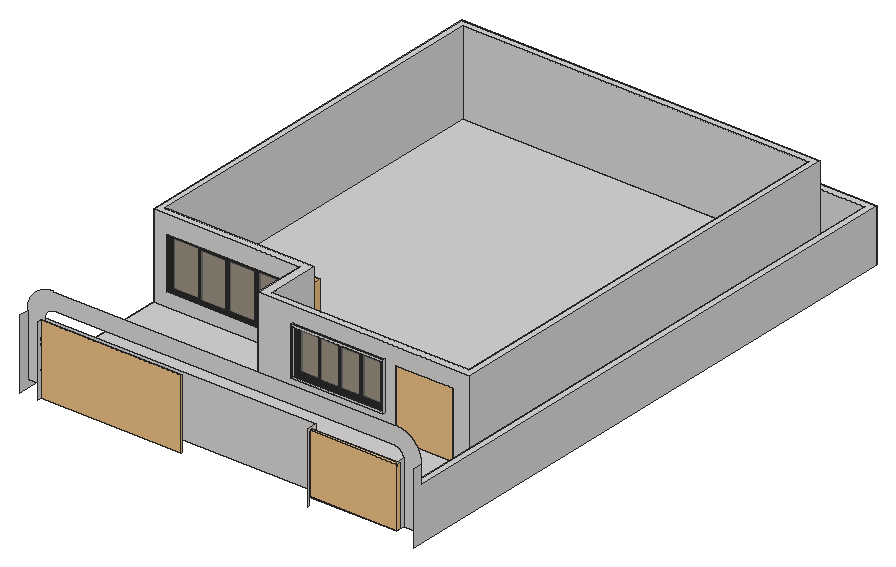
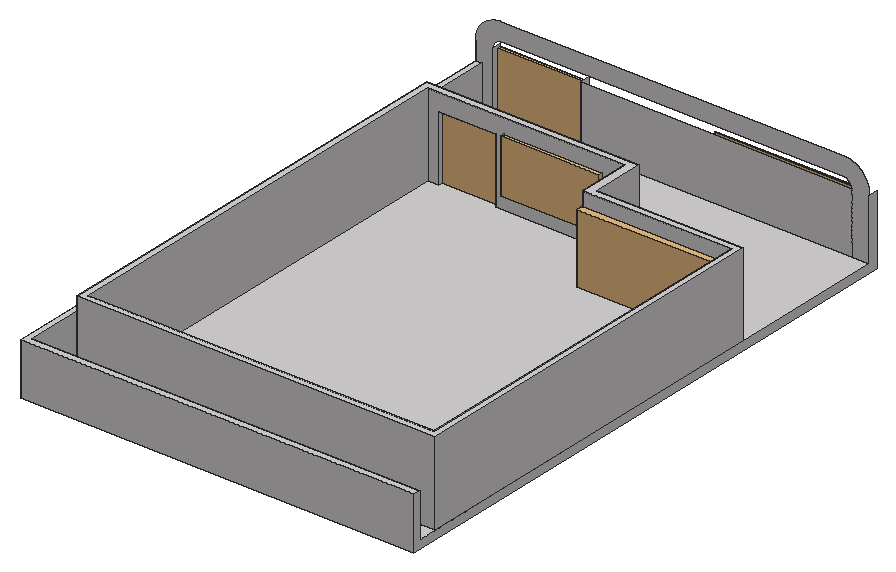
# SketchUp Ruby script. Lengths in inches.
U = 1.inch
M = Sketchup.active_model
def pt(a) = Geom::Point3d.new(a.map { |v| v * U })
def face(e, loops, mat)
  f = e.add_face(loops[0].map { |a| pt(a) })
  loops[1..].each { |l| e.add_face(l.map { |a| pt(a) }).erase! }
  f.material = f.back_material = mat if mat
  f
end
# faces: each face lists its corners as indices into pts; further lists are holes
def faces(e, pts, list, mat = nil) = list.each { |f| face(e, (f[0].is_a?(Array) ? f : [f]).map { |l| l.map { |i| pts[i] } }, mat) }
# xy, xz, yz: faces in a plane at the given z, y or x. An outline is a flat list of corners, or four numbers for a rectangle; further outlines are holes
def ring(l) = l.size == 4 ? [[l[0], l[1]], [l[2], l[1]], [l[2], l[3]], [l[0], l[3]]] : l.each_slice(2).to_a
def flat(e, list, mat, &to3) = list.each { |f| face(e, (f[0].is_a?(Array) ? f : [f]).map { |l| ring(l).map { |u, v| to3.(u, v) } }, mat) }
def xy(e, z, list, mat = nil) = flat(e, list, mat) { |x, y| [x, y, z] }
def xz(e, y, list, mat = nil) = flat(e, list, mat) { |x, z| [x, y, z] }
def yz(e, x, list, mat = nil) = flat(e, list, mat) { |y, z| [x, y, z] }
def lines(e, pts, list) = list.each { |a, b| e.add_line(pt(pts[a]), pt(pts[b])) }
# prism: a flat outline (further loops are holes) pulled along v
def prism(e, loops, v, mat = nil)
  f = face(e, loops, mat); d = Geom::Vector3d.new(v.map { |x| x * U })
  f.pushpull(f.normal.samedirection?(d) ? d.length : -d.length)
end
def box(e, o, s, mat = nil) = prism(e, [[o, [o[0] + s[0], o[1], o[2]], [o[0] + s[0], o[1] + s[1], o[2]], [o[0], o[1] + s[1], o[2]]]], [0, 0, s[2]], mat)
def at(x, y, z, deg = 0) = Geom::Transformation.translation(pt([x, y, z])) * Geom::Transformation.rotation(ORIGIN, Z_AXIS, deg.degrees)
def axes(o, x, y, z) = Geom::Transformation.new([*x, 0, *y, 0, *z, 0, *pt(o).to_a, 1])
def part(name) = M.definitions.add(name)
# library, detail: a bought-in or finely detailed component or shape, given as its bounding box
def library(name, o, s) = part(name).tap { |d| box(d.entities, o, s) }
def detail(e, o, s) = box(e.add_group.entities, o, s)
def put(e, d, t, mat = nil) = e.add_instance(d, t).tap { |i| i.material = mat if mat }
def group(e, t, mat = nil) = e.add_group.tap { |g| g.transformation = t; g.material = mat if mat }.entities
root = M.entities
M.materials.add("T METAL").color = [42, 41, 39]
M.materials.add("[Quartz Light Brown]").color = [215, 212, 212]
M.materials.add("[Terrazzo Tile Light]").color = [219, 217, 210]
M.materials.add("[Translucent_Glass_Gray]").color = [128, 128, 128]
M.materials["[Translucent_Glass_Gray]"].alpha = 0.5
M.materials.add("[Wood Cherry Original]").color = [152, 86, 42]
c1 = library("cong+trinh+1",[72.29,25.93,6.78],[125.98,5.19,98.43])
c2 = library("Group\#56",[0,-0.5,0],[192,0.5,96])
c3 = library("Garniza_zaclona",[1.52,0,0],[127.96,8.15,78.72])
c4 = part("Window frame")
prism(c4.entities,[[[0,70.87,0],[0,0,0],[0,0,47.24],[0,70.87,47.24]],[[0,1.97,1.97],[0,68.9,1.97],[0,68.9,45.28],[0,1.97,45.28]]],[7.875,0,0])
c5 = part("Window sash")
xy(c5.entities,0,[[0,0,3.9375,16.73]])
xy(c5.entities,0.98,[[0,0.98,1.77,15.75],[1.77,0.98,2.85,15.75],[2.85,0.98,3.9375,15.75]])
xy(c5.entities,42.32,[[0,0.98,1.77,15.75],[1.77,0.98,2.85,15.75],[2.85,0.98,3.9375,15.75]])
xy(c5.entities,43.31,[[0,0,3.9375,16.73]])
xz(c5.entities,0,[[0,0,3.9375,43.31]])
xz(c5.entities,0.98,[[0,0.98,1.77,42.32],[1.77,0.98,2.85,42.32],[2.85,0.98,3.9375,42.32]])
xz(c5.entities,15.75,[[0,0.98,1.77,42.32],[1.77,0.98,2.85,42.32],[2.85,0.98,3.9375,42.32]])
xz(c5.entities,16.73,[[0,0,3.9375,43.31]])
yz(c5.entities,0,[[[0,0,16.73,43.31],[0.98,0.98,15.75,42.32]]])
yz(c5.entities,1.77,[[0.98,0.98,15.75,42.32]],"[Translucent_Glass_Gray]")
yz(c5.entities,2.85,[[0.98,0.98,15.75,42.32]],"[Translucent_Glass_Gray]")
yz(c5.entities,3.9375,[[[0,0,16.73,43.31],[0.98,0.98,15.75,42.32]]])
c6 = part("simple+window")
p = [[0,68.9,1.97],[0,35.43,1.97]]
lines(c6.entities,p,[[0,1]])
put(c6.entities,c4,at(0,0,0))
put(c6.entities,c5,axes([1.14,52.17,1.97],[0.71,0,0],[0,1,0],[0,0,1]))
put(c6.entities,c5,axes([1.14,1.97,1.97],[0.71,0,0],[0,1,0],[0,0,1]))
put(c6.entities,c5,axes([3.9375,18.7,1.97],[0.71,0,0],[0,1,0],[0,0,1]))
put(c6.entities,c5,axes([3.9375,35.43,1.97],[0.71,0,0],[0,1,0],[0,0,1]))
c7 = library("Elegant door(double)",[38.88,29.07,0],[76.71,4.33,84.81])
c8 = library("SHOWER+CURTAIN",[-76.11,-2.58,2.78],[135.11,4.99,73.24])
xy(root,0,[[396,38,516,38,516,50,531,50,531,821,0,821,0,50,396,50]],"[Quartz Light Brown]")
xy(root,60,[[531,50,540,50,540,830,0,830,0,821,531,821]],"[Quartz Light Brown]")
xz(root,44,[[24,-12,216,84]],"[Quartz Light Brown]")
xz(root,50,[[0,0,0,84.57,0.03,85.41,0.04,85.7,0.05,85.98,0.11,86.82,0.13,87.11,0.16,87.39,0.1875,87.67,0.22,87.95,0.28,88.51,0.44,89.63,0.49,89.91,0.54,90.1875,0.59,90.47,0.64,90.75,0.69,91.02,0.81,91.58,0.87,91.85,0.93,92.13,0.99,92.4,1.0625,92.68,1.2,93.23,1.28,93.5,1.35,93.77,1.51,94.31,1.59,94.59,1.68,94.86,1.76,95.125,1.85,95.39,2.03,95.93,2.13,96.19,2.23,96.46,2.32,96.73,2.42,96.99,2.53,97.25,2.63,97.51,2.74,97.78,3.07,98.56,3.1875,98.81,3.31,99.07,3.43,99.33,3.55,99.58,3.67,99.84,3.8,100.09,3.92,100.34,4.05,100.6,4.18,100.85,4.32,101.09,4.45,101.34,4.73,101.84,4.87,102.08,5.01,102.33,5.16,102.57,5.3,102.81,5.6,103.29,5.76,103.53,5.91,103.76,6.23,104.24,6.38,104.47,6.55,104.7,6.71,104.93,7.04,105.39,7.21,105.62,7.55,106.06,7.73,106.29,7.9,106.51,8.26,106.95,8.44,107.16,8.625,107.38,8.81,107.59,9,107.81,9.18,108.02,9.375,108.23,9.5625,108.4375,9.76,108.64,9.95,108.85,10.15,109.05,10.35,109.26,10.54,109.46,10.74,109.65,10.95,109.85,11.15,110.05,11.36,110.24,11.5625,110.4375,11.77,110.625,11.98,110.82,12.19,111,12.41,111.19,12.62,111.375,12.84,111.56,13.05,111.74,13.49,112.1,13.71,112.27,13.94,112.45,14.38,112.79,14.61,112.96,15.07,113.29,15.3,113.45,15.53,113.62,15.76,113.77,16.24,114.09,16.47,114.24,16.71,114.4,17.19,114.7,17.43,114.84,17.67,114.99,17.92,115.13,18.16,115.27,18.66,115.55,18.91,115.68,19.15,115.82,19.4,115.95,19.66,116.08,19.91,116.2,20.16,116.33,20.42,116.45,20.67,116.57,20.93,116.69,21.19,116.8125,21.44,116.93,22.22,117.26,22.49,117.37,22.75,117.47,23.01,117.58,23.27,117.68,23.54,117.77,23.81,117.87,24.07,117.97,24.61,118.15,24.875,118.24,25.14,118.32,25.41,118.41,25.69,118.49,26.23,118.65,26.5,118.72,26.77,118.8,27.32,118.9375,27.6,119.01,27.87,119.07,28.15,119.13,28.42,119.19,28.98,119.31,29.25,119.36,29.53,119.41,29.8125,119.46,30.09,119.51,30.37,119.56,31.49,119.72,32.05,119.78,32.33,119.8125,32.61,119.84,32.89,119.87,33.18,119.89,34.02,119.95,34.3,119.96,34.59,119.97,35.43,120,504.57,120,505.41,119.97,505.7,119.96,505.98,119.95,506.82,119.89,507.11,119.87,507.39,119.84,507.67,119.8125,507.95,119.78,508.51,119.72,509.63,119.56,509.91,119.51,510.1875,119.46,510.47,119.41,510.75,119.36,511.02,119.31,511.58,119.19,511.85,119.13,512.13,119.07,512.4,119.01,512.68,118.9375,513.23,118.8,513.5,118.72,513.77,118.65,514.31,118.49,514.59,118.41,514.86,118.32,515.125,118.24,515.39,118.15,515.93,117.97,516.19,117.87,516.46,117.77,516.73,117.68,516.99,117.58,517.25,117.47,517.51,117.37,517.78,117.26,518.56,116.93,518.81,116.8125,519.07,116.69,519.33,116.57,519.58,116.45,519.84,116.33,520.09,116.2,520.34,116.08,520.6,115.95,520.85,115.82,521.09,115.68,521.34,115.55,521.84,115.27,522.08,115.13,522.33,114.99,522.57,114.84,522.81,114.7,523.29,114.4,523.53,114.24,523.76,114.09,524.24,113.77,524.47,113.62,524.7,113.45,524.93,113.29,525.39,112.96,525.62,112.79,526.06,112.45,526.29,112.27,526.51,112.1,526.95,111.74,527.16,111.56,527.38,111.375,527.59,111.19,527.81,111,528.02,110.82,528.23,110.625,528.4375,110.4375,528.64,110.24,528.85,110.05,529.05,109.85,529.26,109.65,529.46,109.46,529.65,109.26,529.85,109.05,530.05,108.85,530.24,108.64,530.4375,108.4375,530.625,108.23,530.82,108.02,531,107.81,531.19,107.59,531.375,107.38,531.56,107.16,531.74,106.95,532.1,106.51,532.27,106.29,532.45,106.06,532.79,105.62,532.96,105.39,533.29,104.93,533.45,104.7,533.62,104.47,533.77,104.24,534.09,103.76,534.24,103.53,534.4,103.29,534.7,102.81,534.84,102.57,534.99,102.33,535.13,102.08,535.27,101.84,535.55,101.34,535.68,101.09,535.82,100.85,535.95,100.6,536.08,100.34,536.2,100.09,536.33,99.84,536.45,99.58,536.57,99.33,536.69,99.07,536.8125,98.81,536.93,98.56,537.26,97.78,537.37,97.51,537.47,97.25,537.58,96.99,537.68,96.73,537.77,96.46,537.87,96.19,537.97,95.93,538.15,95.39,538.24,95.125,538.32,94.86,538.41,94.59,538.49,94.31,538.65,93.77,538.72,93.5,538.8,93.23,538.9375,92.68,539.01,92.4,539.07,92.13,539.13,91.85,539.19,91.58,539.31,91.02,539.36,90.75,539.41,90.47,539.46,90.1875,539.51,89.91,539.56,89.63,539.72,88.51,539.78,87.95,539.8125,87.67,539.84,87.39,539.87,87.11,539.89,86.82,539.95,85.98,539.96,85.7,539.97,85.41,540,84.57,540,60,531,60,531,0,516,0,516,84.28,515.99,84.375,515.99,84.57,515.98,84.66,515.98,84.75,515.97,84.85,515.96,84.94,515.96,85.04,515.95,85.13,515.9375,85.22,515.93,85.32,515.91,85.5,515.89,85.6,515.87,85.78,515.85,85.88,515.84,85.97,515.82,86.0625,515.8,86.16,515.79,86.25,515.75,86.43,515.73,86.53,515.65,86.89,515.62,86.98,515.6,87.08,515.57,87.17,515.55,87.26,515.52,87.35,515.5,87.4375,515.47,87.53,515.32,87.98,515.29,88.06,515.23,88.24,515.19,88.33,515.16,88.42,515.12,88.5,515.09,88.59,515.01,88.77,514.98,88.85,514.9375,88.9375,514.9,89.02,514.86,89.11,514.82,89.19,514.78,89.28,514.73,89.36,514.69,89.45,514.65,89.53,514.61,89.62,514.5625,89.7,514.52,89.78,514.47,89.86,514.42,89.95,514.33,90.11,514.28,90.1875,514.23,90.27,513.98,90.67,513.92,90.75,513.87,90.82,513.82,90.9,513.76,90.98,513.71,91.05,513.65,91.13,513.6,91.21,513.48,91.35,513.42,91.43,513.37,91.5,513.31,91.58,513.25,91.65,513.0625,91.86,513,91.9375,512.9375,92.01,512.8125,92.15,512.75,92.21,512.68,92.28,512.62,92.35,512.55,92.42,512.49,92.49,512.42,92.55,512.35,92.62,512.28,92.68,512.21,92.75,512.15,92.8125,512.01,92.9375,511.9375,93,511.86,93.0625,511.65,93.25,511.58,93.31,511.5,93.37,511.43,93.42,511.35,93.48,511.21,93.6,511.13,93.65,511.05,93.71,510.98,93.76,510.9,93.82,510.82,93.87,510.75,93.92,510.67,93.98,510.27,94.23,510.1875,94.28,510.11,94.33,509.95,94.42,509.86,94.47,509.78,94.52,509.7,94.5625,509.62,94.61,509.53,94.65,509.45,94.69,509.36,94.73,509.28,94.78,509.19,94.82,509.11,94.86,509.02,94.9,508.9375,94.9375,508.85,94.98,508.77,95.01,508.59,95.09,508.5,95.12,508.42,95.16,508.33,95.19,508.24,95.23,508.06,95.29,507.98,95.32,507.53,95.47,507.4375,95.5,507.35,95.52,507.26,95.55,507.17,95.57,507.08,95.6,506.98,95.62,506.89,95.65,506.53,95.73,506.43,95.75,506.25,95.79,506.16,95.8,506.0625,95.82,505.97,95.84,505.88,95.85,505.78,95.87,505.6,95.89,505.5,95.91,505.32,95.93,505.22,95.9375,505.13,95.95,505.04,95.96,504.94,95.96,504.85,95.97,504.75,95.98,504.66,95.98,504.57,95.99,504.375,95.99,504.28,96,35.72,96,35.625,95.99,35.43,95.99,35.34,95.98,35.25,95.98,35.15,95.97,35.06,95.96,34.96,95.96,34.87,95.95,34.78,95.9375,34.68,95.93,34.5,95.91,34.4,95.89,34.22,95.87,34.12,95.85,34.03,95.84,33.9375,95.82,33.84,95.8,33.75,95.79,33.57,95.75,33.47,95.73,33.11,95.65,33.02,95.62,32.92,95.6,32.83,95.57,32.74,95.55,32.65,95.52,32.5625,95.5,32.47,95.47,32.02,95.32,31.94,95.29,31.76,95.23,31.67,95.19,31.58,95.16,31.5,95.12,31.41,95.09,31.23,95.01,31.15,94.98,31.0625,94.9375,30.98,94.9,30.89,94.86,30.81,94.82,30.72,94.78,30.64,94.73,30.55,94.69,30.47,94.65,30.38,94.61,30.3,94.5625,30.22,94.52,30.14,94.47,30.05,94.42,29.89,94.33,29.8125,94.28,29.73,94.23,29.33,93.98,29.25,93.92,29.18,93.87,29.1,93.82,29.02,93.76,28.95,93.71,28.87,93.65,28.79,93.6,28.65,93.48,28.57,93.42,28.5,93.37,28.42,93.31,28.35,93.25,28.14,93.0625,28.0625,93,27.99,92.9375,27.85,92.8125,27.79,92.75,27.72,92.68,27.65,92.62,27.58,92.55,27.51,92.49,27.45,92.42,27.38,92.35,27.32,92.28,27.25,92.21,27.1875,92.15,27.0625,92.01,27,91.9375,26.9375,91.86,26.75,91.65,26.69,91.58,26.63,91.5,26.58,91.43,26.52,91.35,26.4,91.21,26.35,91.13,26.29,91.05,26.24,90.98,26.18,90.9,26.13,90.82,26.08,90.75,26.02,90.67,25.77,90.27,25.72,90.1875,25.67,90.11,25.58,89.95,25.53,89.86,25.48,89.78,25.4375,89.7,25.39,89.62,25.35,89.53,25.31,89.45,25.27,89.36,25.22,89.28,25.18,89.19,25.14,89.11,25.1,89.02,25.0625,88.9375,25.02,88.85,24.99,88.77,24.91,88.59,24.88,88.5,24.84,88.42,24.81,88.33,24.77,88.24,24.71,88.06,24.68,87.98,24.53,87.53,24.5,87.4375,24.48,87.35,24.45,87.26,24.43,87.17,24.4,87.08,24.38,86.98,24.35,86.89,24.27,86.53,24.25,86.43,24.21,86.25,24.2,86.16,24.18,86.0625,24.16,85.97,24.15,85.88,24.13,85.78,24.11,85.6,24.09,85.5,24.07,85.32,24.0625,85.22,24.05,85.13,24.04,85.04,24.04,84.94,24.03,84.85,24.02,84.75,24.02,84.66,24.01,84.57,24.01,84.375,24,84.28,24,0],[24,0,396,84]],"[Quartz Light Brown]")
xz(root,821,[[0,0,531,60]],"[Quartz Light Brown]")
xz(root,830,[[0,-12,540,60]],"[Quartz Light Brown]")
yz(root,0,[[38,-12,38,84,50,84,50,0,821,0,821,60,830,60,830,-12]],"[Quartz Light Brown]")
yz(root,24,[[38,-12,44,84]],"[Quartz Light Brown]")
yz(root,396,[[36,-12,38,-12,38,0,50,0,50,84,36,84]],"[Terrazzo Tile Light]")
yz(root,516,[[38,0,50,84]],"[Quartz Light Brown]")
yz(root,531,[[50,0,821,60]],"[Quartz Light Brown]")
yz(root,540,[[38,-12,830,-12,830,60,50,60,50,84,38,84]],"[Quartz Light Brown]")
put(root,c1,axes([327.15,16.74,-5.59],[0.9525,0,0],[0,0.85,0],[0,0,0.8245]),"[Quartz Light Brown]")
put(root,c2,at(24,44,-12),"[Wood Cherry Original]")
put(root,c3,axes([9,275,0],[1.58151,0,0],[0,1.1771,0],[0,0,1.20432]),"[Quartz Light Brown]")
g1 = group(root,at(0,194,0),"[Quartz Light Brown]")
xy(g1,0,[[201,0,201,72,0,72,0,600,492,600,492,0,468,0,468,9,483,9,483,591,9,591,9,81,213,81,213,9,390,9,390,0]])
xy(g1,18,[[18,72,183,81]])
xy(g1,27,[[249,-3,375,0]])
xy(g1,29.5,[[251.5,-3,372.5,0]])
xy(g1,30,[[252,0,372,9]])
xy(g1,90,[[252,0,372,9],[390,0,468,9],[18,72,183,81]])
xy(g1,90.5,[[251.5,-3,372.5,0]])
xy(g1,93,[[249,-3,375,0]])
xy(g1,114,[[[201,0,492,0,492,600,0,600,0,72,201,72],[213,9,213,81,9,81,9,591,483,591,483,9]]])
xz(g1,-3,[[[249,27,375,93],[251.5,29.5,372.5,90.5]]])
xz(g1,0,[[[201,0,390,0,390,90,468,90,468,0,492,0,492,114,201,114],[249,27,375,93]],[[251.5,29.5,372.5,90.5],[252,30,372,90]],[372.5,29.5,373,91.5],[373,29.5,373.5,91.5]])
xz(g1,9,[[[213,0,213,114,483,114,483,0,468,0,468,90,390,90,390,0],[252,30,372,90]]])
xz(g1,72,[[[0,0,201,114],[18,18,183,90]]])
xz(g1,81,[[[9,0,213,114],[18,18,183,90]]])
xz(g1,591,[[9,0,483,114]])
xz(g1,600,[[0,0,492,114]])
yz(g1,0,[[72,0,600,114]])
yz(g1,9,[[81,0,591,114]])
yz(g1,18,[[72,18,81,90]])
yz(g1,183,[[72,18,81,90]])
yz(g1,201,[[0,0,72,114]])
yz(g1,213,[[9,0,81,114]])
yz(g1,249,[[-3,27,0,93]])
yz(g1,251.5,[[-3,29.5,0,90.5]])
yz(g1,252,[[0,30,9,90]])
yz(g1,372,[[0,30,9,90]])
yz(g1,372.5,[[-3,29.5,0,90.5]])
yz(g1,375,[[-3,27,0,93]])
yz(g1,390,[[0,0,9,90]])
yz(g1,468,[[0,0,9,90]])
yz(g1,483,[[9,0,591,114]])
yz(g1,492,[[0,0,600,114]])
put(g1,c6,axes([252,5.01,30],[0,-0.5,0],[1.69333,0,0],[0,0,1.27]),"T METAL")
put(g1,c7,axes([350.47,-29.07,0],[1.01686,0,0],[0,1,0],[0,0,1.0612]))
put(g1,c6,axes([18,77.01,18],[0,-0.5,0],[2.32833,0,0],[0,0,1.524]),"T METAL")
put(g1,c8,at(319.92,11.58,17.23))
